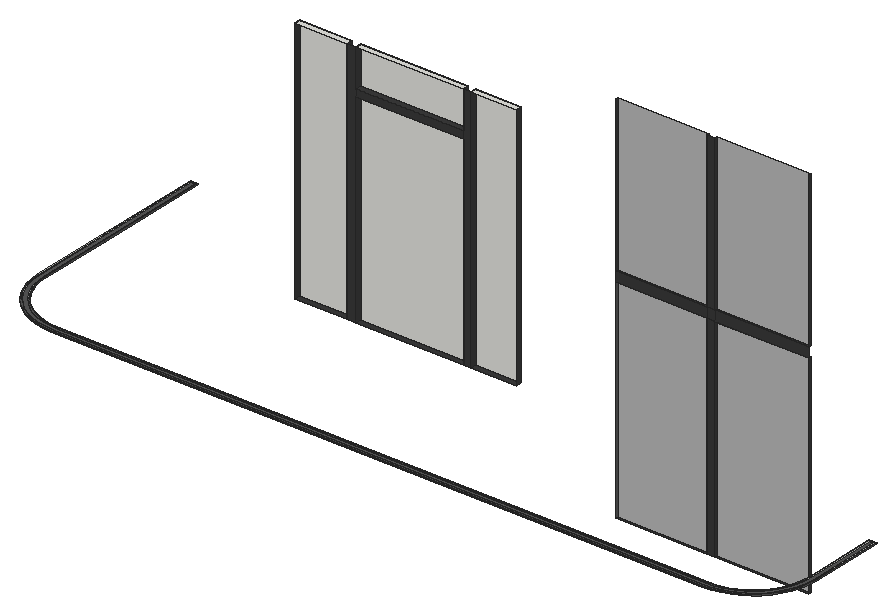
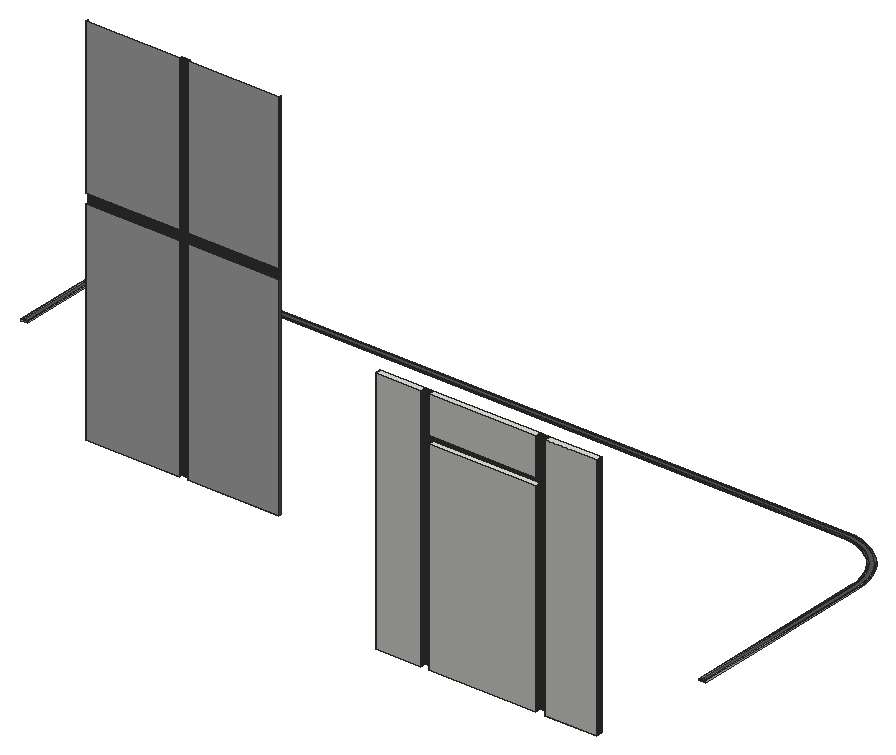
# SketchUp Ruby script. Lengths in inches.
U = 1.inch
M = Sketchup.active_model
def pt(a) = Geom::Point3d.new(a.map { |v| v * U })
def face(e, loops, mat)
  f = e.add_face(loops[0].map { |a| pt(a) })
  loops[1..].each { |l| e.add_face(l.map { |a| pt(a) }).erase! }
  f.material = f.back_material = mat if mat
  f
end
# faces: each face lists its corners as indices into pts; further lists are holes
def faces(e, pts, list, mat = nil) = list.each { |f| face(e, (f[0].is_a?(Array) ? f : [f]).map { |l| l.map { |i| pts[i] } }, mat) }
# xy, xz, yz: faces in a plane at the given z, y or x. An outline is a flat list of corners, or four numbers for a rectangle; further outlines are holes
def ring(l) = l.size == 4 ? [[l[0], l[1]], [l[2], l[1]], [l[2], l[3]], [l[0], l[3]]] : l.each_slice(2).to_a
def flat(e, list, mat, &to3) = list.each { |f| face(e, (f[0].is_a?(Array) ? f : [f]).map { |l| ring(l).map { |u, v| to3.(u, v) } }, mat) }
def xy(e, z, list, mat = nil) = flat(e, list, mat) { |x, y| [x, y, z] }
def xz(e, y, list, mat = nil) = flat(e, list, mat) { |x, z| [x, y, z] }
def yz(e, x, list, mat = nil) = flat(e, list, mat) { |y, z| [x, y, z] }
def lines(e, pts, list) = list.each { |a, b| e.add_line(pt(pts[a]), pt(pts[b])) }
# prism: a flat outline (further loops are holes) pulled along v
def prism(e, loops, v, mat = nil)
  f = face(e, loops, mat); d = Geom::Vector3d.new(v.map { |x| x * U })
  f.pushpull(f.normal.samedirection?(d) ? d.length : -d.length)
end
def box(e, o, s, mat = nil) = prism(e, [[o, [o[0] + s[0], o[1], o[2]], [o[0] + s[0], o[1] + s[1], o[2]], [o[0], o[1] + s[1], o[2]]]], [0, 0, s[2]], mat)
def at(x, y, z, deg = 0) = Geom::Transformation.translation(pt([x, y, z])) * Geom::Transformation.rotation(ORIGIN, Z_AXIS, deg.degrees)
def axes(o, x, y, z) = Geom::Transformation.new([*x, 0, *y, 0, *z, 0, *pt(o).to_a, 1])
def part(name) = M.definitions.add(name)
# library, detail: a bought-in or finely detailed component or shape, given as its bounding box
def library(name, o, s) = part(name).tap { |d| box(d.entities, o, s) }
def detail(e, o, s) = box(e.add_group.entities, o, s)
def put(e, d, t, mat = nil) = e.add_instance(d, t).tap { |i| i.material = mat if mat }
def group(e, t, mat = nil) = e.add_group.tap { |g| g.transformation = t; g.material = mat if mat }.entities
root = M.entities
M.materials.add("[Color M06]").color = [86, 86, 86]
M.materials.add("[Color M07]").color = [58, 58, 58]
M.materials.add("[Mirror 01]").color = [185, 185, 185]
xy(root,145.24,[[403.41,90.75,440.73,91.75],[444.31,90.75,482.61,91.75]],"[Color M07]")
xy(root,145.37,[[233.89,138.25,255.22,140.6875],[259.01,138.25,303.08,140.6875],[306,138.25,324.79,140.6875]],"[Color M07]")
xy(root,176.0625,[[220.41,30.65,217.06,30.87,213.78,31.52,210.61,32.6,207.6,34.08,204.82,35.9375,202.3,38.15,200.09,40.66,198.23,43.45,196.75,46.45,195.68,49.625,195.02,52.91,194.8,56.25,194.8,133.75,196.73,133.75,196.73,56.25,196.9375,53.16,197.54,50.12,198.54,47.19,199.9,44.41,201.625,41.84,203.67,39.51,206,37.47,208.57,35.75,211.35,34.38,214.28,33.38,217.32,32.78,220.41,32.58,487.41,32.58,490.5,32.78,493.53,33.38,496.47,34.38,499.24,35.75,501.82,37.47,504.15,39.51,506.1875,41.84,507.91,44.41,509.28,47.19,510.27,50.12,510.88,53.16,511.08,56.25,511.08,86.25,513.01,86.25,513.01,56.25,512.79,52.91,512.14,49.625,511.0625,46.45,509.58,43.45,507.72,40.66,505.51,38.15,502.99,35.9375,500.21,34.08,497.2,32.6,494.03,31.52,490.75,30.87,487.41,30.65]])
xy(root,176.0625,[[[220.41,30.12,217,30.34,213.64,31.01,210.41,32.11,207.34,33.62,204.5,35.52,201.93,37.77,199.68,40.34,197.78,43.1875,196.27,46.25,195.17,49.49,194.5,52.84,194.28,56.25,194.28,134.28,197.26,134.28,197.26,56.25,197.46,53.23,198.05,50.26,199.02,47.39,200.36,44.68,202.04,42.16,204.04,39.88,206.31,37.89,208.83,36.2,211.55,34.86,214.42,33.89,217.39,33.3,220.41,33.1,487.41,33.1,490.43,33.3,493.4,33.89,496.27,34.86,498.98,36.2,501.5,37.89,503.78,39.88,505.77,42.16,507.45,44.68,508.79,47.39,509.77,50.26,510.36,53.23,510.56,56.25,510.56,86.78,513.54,86.78,513.54,56.25,513.3125,52.84,512.65,49.49,511.55,46.25,510.04,43.1875,508.14,40.34,505.88,37.77,503.3125,35.52,500.47,33.62,497.41,32.11,494.17,31.01,490.82,30.34,487.41,30.12],[220.41,30.65,487.41,30.65,490.75,30.87,494.03,31.52,497.2,32.6,500.21,34.08,502.99,35.9375,505.51,38.15,507.72,40.66,509.58,43.45,511.0625,46.45,512.14,49.625,512.79,52.91,513.01,56.25,513.01,86.25,511.08,86.25,511.08,56.25,510.88,53.16,510.27,50.12,509.28,47.19,507.91,44.41,506.1875,41.84,504.15,39.51,501.82,37.47,499.24,35.75,496.47,34.38,493.53,33.38,490.5,32.78,487.41,32.58,220.41,32.58,217.32,32.78,214.28,33.38,211.35,34.38,208.57,35.75,206,37.47,203.67,39.51,201.625,41.84,199.9,44.41,198.54,47.19,197.54,50.12,196.9375,53.16,196.73,56.25,196.73,133.75,194.8,133.75,194.8,56.25,195.02,52.91,195.68,49.625,196.75,46.45,198.23,43.45,200.09,40.66,202.3,38.15,204.82,35.9375,207.6,34.08,210.61,32.6,213.78,31.52,217.06,30.87]]],"[Color M06]")
xy(root,176.5,[[[220.41,30.12,487.41,30.12,490.82,30.34,494.17,31.01,497.41,32.11,500.47,33.62,503.3125,35.52,505.88,37.77,508.14,40.34,510.04,43.1875,511.55,46.25,512.65,49.49,513.3125,52.84,513.54,56.25,513.54,86.78,510.56,86.78,510.56,56.25,510.36,53.23,509.77,50.26,508.79,47.39,507.45,44.68,505.77,42.16,503.78,39.88,501.5,37.89,498.98,36.2,496.27,34.86,493.4,33.89,490.43,33.3,487.41,33.1,220.41,33.1,217.39,33.3,214.42,33.89,211.55,34.86,208.83,36.2,206.31,37.89,204.04,39.88,202.04,42.16,200.36,44.68,199.02,47.39,198.05,50.26,197.46,53.23,197.26,56.25,197.26,134.28,194.28,134.28,194.28,56.25,194.5,52.84,195.17,49.49,196.27,46.25,197.78,43.1875,199.68,40.34,201.93,37.77,204.5,35.52,207.34,33.62,210.41,32.11,213.64,31.01,217,30.34],[220.41,30.65,217.06,30.87,213.78,31.52,210.61,32.6,207.6,34.08,204.82,35.9375,202.3,38.15,200.09,40.66,198.23,43.45,196.75,46.45,195.68,49.625,195.02,52.91,194.8,56.25,194.8,133.75,196.73,133.75,196.73,56.25,196.9375,53.16,197.54,50.12,198.54,47.19,199.9,44.41,201.625,41.84,203.67,39.51,206,37.47,208.57,35.75,211.35,34.38,214.28,33.38,217.32,32.78,220.41,32.58,487.41,32.58,490.5,32.78,493.53,33.38,496.47,34.38,499.24,35.75,501.82,37.47,504.15,39.51,506.1875,41.84,507.91,44.41,509.28,47.19,510.27,50.12,510.88,53.16,511.08,56.25,511.08,86.25,513.01,86.25,513.01,56.25,512.79,52.91,512.14,49.625,511.0625,46.45,509.58,43.45,507.72,40.66,505.51,38.15,502.99,35.9375,500.21,34.08,497.2,32.6,494.03,31.52,490.75,30.87,487.41,30.65]],[220.41,30.65,487.41,30.65,490.75,30.87,494.03,31.52,497.2,32.6,500.21,34.08,502.99,35.9375,505.51,38.15,507.72,40.66,509.58,43.45,511.0625,46.45,512.14,49.625,512.79,52.91,513.01,56.25,513.01,86.25,511.08,86.25,511.08,56.25,510.88,53.16,510.27,50.12,509.28,47.19,507.91,44.41,506.1875,41.84,504.15,39.51,501.82,37.47,499.24,35.75,496.47,34.38,493.53,33.38,490.5,32.78,487.41,32.58,220.41,32.58,217.32,32.78,214.28,33.38,211.35,34.38,208.57,35.75,206,37.47,203.67,39.51,201.625,41.84,199.9,44.41,198.54,47.19,197.54,50.12,196.9375,53.16,196.73,56.25,196.73,133.75,194.8,133.75,194.8,56.25,195.02,52.91,195.68,49.625,196.75,46.45,198.23,43.45,200.09,40.66,202.3,38.15,204.82,35.9375,207.6,34.08,210.61,32.6,213.78,31.52,217.06,30.87]],"[Color M06]")
xy(root,228.29,[[259.01,138.25,303.08,140.6875]])
xy(root,231.45,[[259.01,138.25,303.08,140.6875]],"[Color M07]")
xy(root,231.82,[[403.41,90.75,440.73,91.75],[444.31,90.75,482.61,91.75]],"[Color M07]")
xy(root,235.99,[[403.41,90.75,440.73,91.75],[444.31,90.75,482.61,91.75]],"[Color M07]")
xy(root,246.69,[[233.89,138.25,255.22,140.6875],[259.01,138.25,303.08,140.6875],[306,138.25,324.79,140.6875]])
xz(root,30.12,[[220.41,176.0625,487.41,176.5]],"[Color M06]")
xz(root,30.65,[[220.41,176.0625,487.41,176.5]])
xz(root,32.58,[[220.41,176.0625,487.41,176.5]])
xz(root,33.1,[[220.41,176.0625,487.41,176.5]],"[Color M06]")
xz(root,86.25,[[511.08,176.0625,513.01,176.5]])
xz(root,86.78,[[510.56,176.0625,513.54,176.5]])
xz(root,90.75,[[440.73,145.24,444.31,231.82],[403.41,231.82,440.73,235.99],[440.73,231.82,444.31,235.99],[444.31,231.82,482.61,235.99],[440.73,235.99,444.31,299.08]],"[Color M07]")
xz(root,91.75,[[403.41,145.24,440.73,231.82],[444.31,145.24,482.61,231.82],[403.41,235.99,440.73,299.08],[444.31,235.99,482.61,299.08]],"[Mirror 01]")
xz(root,133.75,[[194.8,176.0625,196.73,176.5]])
xz(root,134.28,[[194.28,176.0625,197.26,176.5]])
xz(root,138.25,[[255.22,145.37,259.01,246.69],[303.08,145.37,306,246.69],[259.01,228.29,303.08,231.45]],"[Color M07]")
xz(root,140.6875,[[233.89,145.37,255.22,246.69],[259.01,145.37,303.08,228.29],[306,145.37,324.79,246.69],[259.01,231.45,303.08,246.69]])
yz(root,194.28,[[56.25,176.0625,86.25,176.5],[86.25,176.0625,95.25,176.5],[95.25,176.0625,134.28,176.5]])
yz(root,194.8,[[56.25,176.0625,86.25,176.5],[86.25,176.0625,95.25,176.5],[95.25,176.0625,133.75,176.5]])
yz(root,196.73,[[56.25,176.0625,86.25,176.5],[86.25,176.0625,133.75,176.5]])
yz(root,197.26,[[56.25,176.0625,86.25,176.5],[86.25,176.0625,134.28,176.5]],"[Color M06]")
yz(root,233.89,[[138.25,145.37,140.6875,246.69]],"[Color M07]")
yz(root,255.22,[[138.25,145.37,140.6875,246.69]],"[Color M07]")
yz(root,259.01,[[138.25,145.37,140.6875,228.29],[138.25,231.45,140.6875,246.69]],"[Color M07]")
yz(root,303.08,[[138.25,145.37,140.6875,228.29],[138.25,231.45,140.6875,246.69]],"[Color M07]")
yz(root,306,[[138.25,145.37,140.6875,246.69]],"[Color M07]")
yz(root,324.79,[[138.25,145.37,140.6875,246.69]],"[Color M07]")
yz(root,403.41,[[90.75,145.24,91.75,231.82]],"[Color M06]")
yz(root,403.41,[[90.75,235.99,91.75,299.08]],"[Color M07]")
yz(root,440.73,[[90.75,145.24,91.75,231.82],[90.75,235.99,91.75,299.08]],"[Color M07]")
yz(root,444.31,[[90.75,145.24,91.75,231.82],[90.75,235.99,91.75,299.08]],"[Color M07]")
yz(root,482.61,[[90.75,145.24,91.75,231.82],[90.75,235.99,91.75,299.08]],"[Color M07]")
yz(root,510.56,[[56.25,176.0625,86.78,176.5]])
yz(root,511.08,[[56.25,176.0625,86.25,176.5]])
yz(root,513.01,[[56.25,176.0625,86.25,176.5]])
yz(root,513.54,[[56.25,176.0625,86.78,176.5]],"[Color M06]")
p = [[217,30.34,176.0625],[220.41,30.12,176.0625],[220.41,30.12,176.5],[217,30.34,176.5],[487.41,30.12,176.0625],[490.82,30.34,176.0625],
  [490.82,30.34,176.5],[487.41,30.12,176.5],[213.64,31.01,176.0625],[213.64,31.01,176.5],[494.17,31.01,176.0625],[494.17,31.01,176.5],
  [220.41,30.65,176.0625],[217.06,30.87,176.0625],[217.06,30.87,176.5],[220.41,30.65,176.5],[490.75,30.87,176.0625],[487.41,30.65,176.0625],
  [487.41,30.65,176.5],[490.75,30.87,176.5],[213.78,31.52,176.0625],[213.78,31.52,176.5],[494.03,31.52,176.0625],[494.03,31.52,176.5],
  [210.41,32.11,176.0625],[210.41,32.11,176.5],[497.41,32.11,176.0625],[497.41,32.11,176.5],[210.61,32.6,176.0625],[210.61,32.6,176.5],
  [497.2,32.6,176.0625],[497.2,32.6,176.5],[207.34,33.62,176.0625],[207.34,33.62,176.5],[500.47,33.62,176.0625],[500.47,33.62,176.5],
  [207.6,34.08,176.0625],[207.6,34.08,176.5],[217.32,32.78,176.0625],[220.41,32.58,176.0625],[220.41,32.58,176.5],[217.32,32.78,176.5],
  [487.41,32.58,176.0625],[490.5,32.78,176.0625],[490.5,32.78,176.5],[487.41,32.58,176.5],[500.21,34.08,176.0625],[500.21,34.08,176.5],
  [214.28,33.38,176.0625],[214.28,33.38,176.5],[493.53,33.38,176.0625],[493.53,33.38,176.5],[220.41,33.1,176.0625],[217.39,33.3,176.0625],
  [217.39,33.3,176.5],[220.41,33.1,176.5],[490.43,33.3,176.0625],[487.41,33.1,176.0625],[487.41,33.1,176.5],[490.43,33.3,176.5],
  [214.42,33.89,176.0625],[214.42,33.89,176.5],[493.4,33.89,176.0625],[493.4,33.89,176.5],[211.35,34.38,176.0625],[211.35,34.38,176.5],
  [496.47,34.38,176.0625],[496.47,34.38,176.5],[204.5,35.52,176.0625],[204.5,35.52,176.5],[503.3125,35.52,176.0625],[503.3125,35.52,176.5],
  [211.55,34.86,176.0625],[211.55,34.86,176.5],[496.27,34.86,176.0625],[496.27,34.86,176.5],[204.82,35.9375,176.0625],[204.82,35.9375,176.5],
  [502.99,35.9375,176.0625],[502.99,35.9375,176.5],[208.57,35.75,176.0625],[208.57,35.75,176.5],[499.24,35.75,176.0625],[499.24,35.75,176.5],
  [208.83,36.2,176.0625],[208.83,36.2,176.5],[498.98,36.2,176.0625],[498.98,36.2,176.5],[201.93,37.77,176.0625],[201.93,37.77,176.5],
  [505.88,37.77,176.0625],[505.88,37.77,176.5],[206,37.47,176.0625],[206,37.47,176.5],[501.82,37.47,176.0625],[501.82,37.47,176.5],
  [202.3,38.15,176.0625],[202.3,38.15,176.5],[505.51,38.15,176.0625],[505.51,38.15,176.5],[206.31,37.89,176.0625],[206.31,37.89,176.5],
  [501.5,37.89,176.0625],[501.5,37.89,176.5],[203.67,39.51,176.0625],[203.67,39.51,176.5],[504.15,39.51,176.0625],[504.15,39.51,176.5],
  [199.68,40.34,176.0625],[199.68,40.34,176.5],[508.14,40.34,176.0625],[508.14,40.34,176.5],[204.04,39.88,176.0625],[204.04,39.88,176.5],
  [503.78,39.88,176.0625],[503.78,39.88,176.5],[200.09,40.66,176.0625],[200.09,40.66,176.5],[507.72,40.66,176.0625],[507.72,40.66,176.5],
  [201.625,41.84,176.0625],[201.625,41.84,176.5],[506.1875,41.84,176.0625],[506.1875,41.84,176.5],[202.04,42.16,176.0625],[202.04,42.16,176.5],
  [505.77,42.16,176.0625],[505.77,42.16,176.5],[197.78,43.1875,176.0625],[197.78,43.1875,176.5],[510.04,43.1875,176.0625],[510.04,43.1875,176.5],
  [198.23,43.45,176.0625],[198.23,43.45,176.5],[509.58,43.45,176.0625],[509.58,43.45,176.5],[199.9,44.41,176.0625],[199.9,44.41,176.5],
  [507.91,44.41,176.0625],[507.91,44.41,176.5],[200.36,44.68,176.0625],[200.36,44.68,176.5],[507.45,44.68,176.0625],[507.45,44.68,176.5],
  [196.27,46.25,176.0625],[196.27,46.25,176.5],[511.55,46.25,176.0625],[511.55,46.25,176.5],[196.75,46.45,176.0625],[196.75,46.45,176.5],
  [511.0625,46.45,176.0625],[511.0625,46.45,176.5],[198.54,47.19,176.0625],[198.54,47.19,176.5],[509.28,47.19,176.0625],[509.28,47.19,176.5],
  [199.02,47.39,176.0625],[199.02,47.39,176.5],[508.79,47.39,176.0625],[508.79,47.39,176.5],[195.17,49.49,176.0625],[195.17,49.49,176.5],
  [512.65,49.49,176.0625],[512.65,49.49,176.5],[195.68,49.625,176.0625],[195.68,49.625,176.5],[512.14,49.625,176.0625],[512.14,49.625,176.5],
  [197.54,50.12,176.0625],[197.54,50.12,176.5],[510.27,50.12,176.0625],[510.27,50.12,176.5],[198.05,50.26,176.0625],[198.05,50.26,176.5],
  [509.77,50.26,176.0625],[509.77,50.26,176.5],[194.5,52.84,176.0625],[194.5,52.84,176.5],[513.3125,52.84,176.0625],[513.3125,52.84,176.5],
  [195.02,52.91,176.0625],[195.02,52.91,176.5],[512.79,52.91,176.0625],[512.79,52.91,176.5],[196.9375,53.16,176.0625],[196.9375,53.16,176.5],
  [510.88,53.16,176.0625],[510.88,53.16,176.5],[197.46,53.23,176.0625],[197.46,53.23,176.5],[510.36,53.23,176.0625],[510.36,53.23,176.5],
  [194.28,56.25,176.0625],[194.28,56.25,176.5],[513.54,56.25,176.0625],[513.54,56.25,176.5],[194.8,56.25,176.0625],[194.8,56.25,176.5],
  [513.01,56.25,176.0625],[513.01,56.25,176.5],[196.73,56.25,176.0625],[196.73,56.25,176.5],[197.26,56.25,176.0625],[197.26,56.25,176.5],
  [510.56,56.25,176.0625],[510.56,56.25,176.5],[511.08,56.25,176.0625],[511.08,56.25,176.5]]
faces(root,p,[[0,1,2,3],[4,5,6,7],[8,0,3,9],[5,10,11,6],[24,8,9,25],[10,26,27,11],[32,24,25,33],[26,34,35,27],
  [52,53,54,55],[56,57,58,59],[53,60,61,54],[62,56,59,63],[68,32,33,69],[34,70,71,35],[60,72,73,61],[74,62,63,75],
  [72,84,85,73],[86,74,75,87],[88,68,69,89],[70,90,91,71],[84,100,101,85],[102,86,87,103],[108,88,89,109],[90,110,111,91],
  [100,112,113,101],[114,102,103,115],[112,124,125,113],[126,114,115,127],[128,108,109,129],[110,130,131,111],[124,140,141,125],[142,126,127,143],
  [144,128,129,145],[130,146,147,131],[140,156,157,141],[158,142,143,159],[160,144,145,161],[146,162,163,147],[156,172,173,157],[174,158,159,175],
  [176,160,161,177],[162,178,179,163],[172,188,189,173],[190,174,175,191],[192,176,177,193],[178,194,195,179],[188,202,203,189],[204,190,191,205]],"[Color M06]")
faces(root,p,[[12,13,14,15],[16,17,18,19],[13,20,21,14],[22,16,19,23],[20,28,29,21],[30,22,23,31],[28,36,37,29],[38,39,40,41],
  [42,43,44,45],[46,30,31,47],[48,38,41,49],[43,50,51,44],[64,48,49,65],[50,66,67,51],[36,76,77,37],[78,46,47,79],
  [80,64,65,81],[66,82,83,67],[92,80,81,93],[82,94,95,83],[76,96,97,77],[98,78,79,99],[104,92,93,105],[94,106,107,95],
  [96,116,117,97],[118,98,99,119],[120,104,105,121],[106,122,123,107],[116,132,133,117],[134,118,119,135],[136,120,121,137],[122,138,139,123],
  [132,148,149,133],[150,134,135,151],[152,136,137,153],[138,154,155,139],[148,164,165,149],[166,150,151,167],[168,152,153,169],[154,170,171,155],
  [164,180,181,165],[182,166,167,183],[184,168,169,185],[170,186,187,171],[180,196,197,181],[198,182,183,199],[200,184,185,201],[186,206,207,187]])
